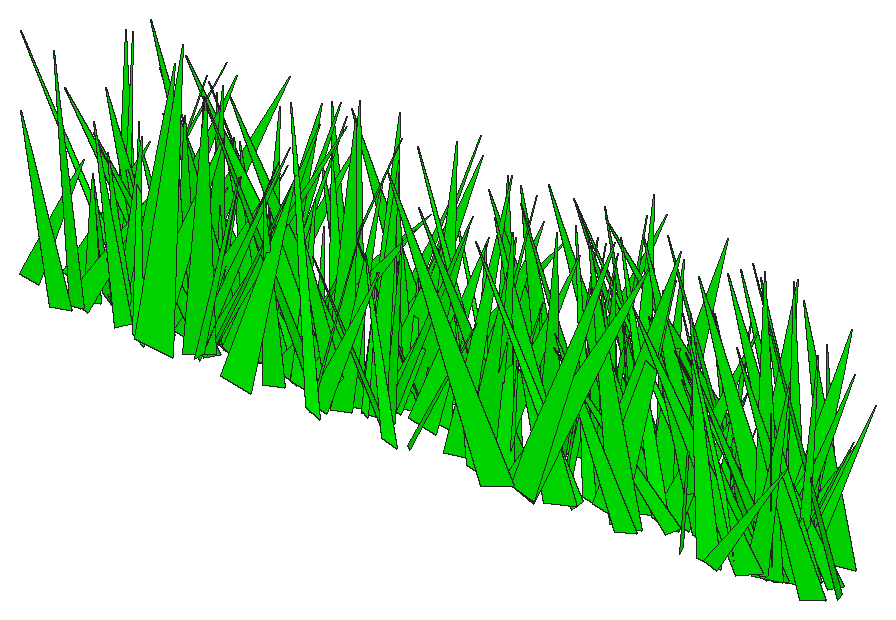
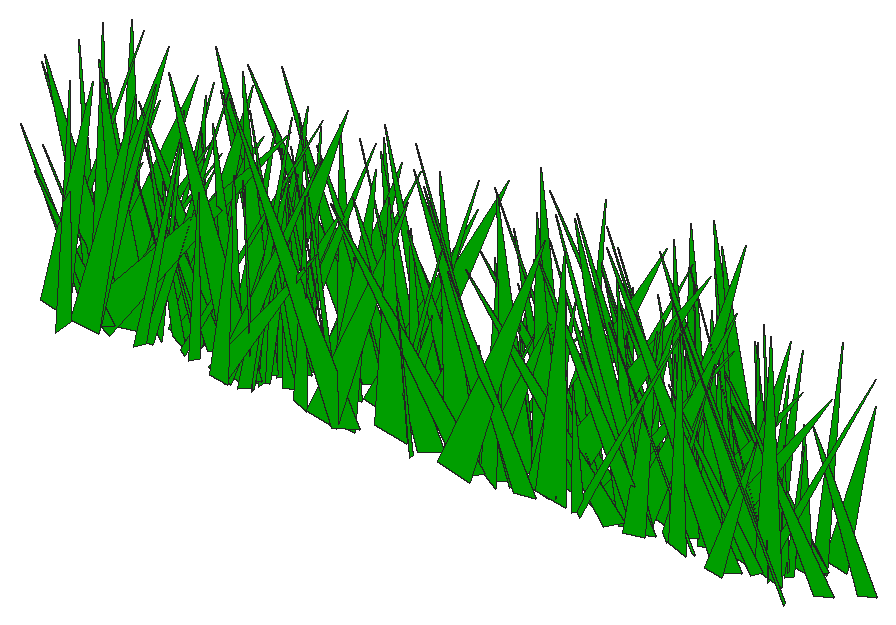
# SketchUp Ruby script. Lengths in inches.
U = 1.inch
M = Sketchup.active_model
def pt(a) = Geom::Point3d.new(a.map { |v| v * U })
def face(e, loops, mat)
  f = e.add_face(loops[0].map { |a| pt(a) })
  loops[1..].each { |l| e.add_face(l.map { |a| pt(a) }).erase! }
  f.material = f.back_material = mat if mat
  f
end
# faces: each face lists its corners as indices into pts; further lists are holes
def faces(e, pts, list, mat = nil) = list.each { |f| face(e, (f[0].is_a?(Array) ? f : [f]).map { |l| l.map { |i| pts[i] } }, mat) }
# xy, xz, yz: faces in a plane at the given z, y or x. An outline is a flat list of corners, or four numbers for a rectangle; further outlines are holes
def ring(l) = l.size == 4 ? [[l[0], l[1]], [l[2], l[1]], [l[2], l[3]], [l[0], l[3]]] : l.each_slice(2).to_a
def flat(e, list, mat, &to3) = list.each { |f| face(e, (f[0].is_a?(Array) ? f : [f]).map { |l| ring(l).map { |u, v| to3.(u, v) } }, mat) }
def xy(e, z, list, mat = nil) = flat(e, list, mat) { |x, y| [x, y, z] }
def xz(e, y, list, mat = nil) = flat(e, list, mat) { |x, z| [x, y, z] }
def yz(e, x, list, mat = nil) = flat(e, list, mat) { |y, z| [x, y, z] }
def lines(e, pts, list) = list.each { |a, b| e.add_line(pt(pts[a]), pt(pts[b])) }
# prism: a flat outline (further loops are holes) pulled along v
def prism(e, loops, v, mat = nil)
  f = face(e, loops, mat); d = Geom::Vector3d.new(v.map { |x| x * U })
  f.pushpull(f.normal.samedirection?(d) ? d.length : -d.length)
end
def box(e, o, s, mat = nil) = prism(e, [[o, [o[0] + s[0], o[1], o[2]], [o[0] + s[0], o[1] + s[1], o[2]], [o[0], o[1] + s[1], o[2]]]], [0, 0, s[2]], mat)
def at(x, y, z, deg = 0) = Geom::Transformation.translation(pt([x, y, z])) * Geom::Transformation.rotation(ORIGIN, Z_AXIS, deg.degrees)
def axes(o, x, y, z) = Geom::Transformation.new([*x, 0, *y, 0, *z, 0, *pt(o).to_a, 1])
def part(name) = M.definitions.add(name)
# library, detail: a bought-in or finely detailed component or shape, given as its bounding box
def library(name, o, s) = part(name).tap { |d| box(d.entities, o, s) }
def detail(e, o, s) = box(e.add_group.entities, o, s)
def put(e, d, t, mat = nil) = e.add_instance(d, t).tap { |i| i.material = mat if mat }
def group(e, t, mat = nil) = e.add_group.tap { |g| g.transformation = t; g.material = mat if mat }.entities
root = M.entities
M.materials.add("[0065_Lime]").color = [0, 255, 0]
c1 = part("fur_instance\#9")
p = [[0.8125,0,1.79],[0.67,-0.02,1.48],[0,-0.11,0],[0,0.11,0]]
faces(c1.entities,p,[[0,1,2,3]])
put(root,c1,axes([46.01,26.64,1.48],[0.39312,0.7455,1.32268],[-5.34892,0.11187,-1.06093],[-1.47663,-0.20675,4.19524]),"[0065_Lime]")
put(root,c1,axes([43.41,27.83,1.48],[1.65186,-0.62517,0.32117],[4.35522,0.21232,-0.97179],[0.99087,0.10897,3.73597]),"[0065_Lime]")
put(root,c1,axes([48.13,28.89,1.48],[-7.52684,0.16689,0.34184],[-1.24991,-1.03405,-1.29256],[0.15794,-0.2299,6.06191]),"[0065_Lime]")
put(root,c1,axes([46.45,27.2,1.48],[5.228,0.61413,2.31199],[-4.08637,0.83396,-1.30923],[-3.23754,-0.0609,5.38591]),"[0065_Lime]")
put(root,c1,axes([44.8125,28.98,1.48],[1.38787,0.72801,0.30258],[-4.98253,0.1713,1.31015],[1.46775,-0.10687,4.16142]),"[0065_Lime]")
put(root,c1,axes([46.98,28.53,1.48],[-3.31547,-0.39766,0.2806],[2.50986,-0.4424,-1.3872],[1.35212,-0.15388,3.26305]),"[0065_Lime]")
put(root,c1,axes([46.74,27.85,1.48],[2.77219,-0.52959,0.05829],[3.63715,0.37908,0.95828],[-0.99022,-0.09025,3.68301]),"[0065_Lime]")
put(root,c1,axes([47.58,29.18,1.48],[3.7097,0.99816,0.96893],[-6.88972,0.54666,-1.41749],[-2.09988,-0.03022,6.36253]),"[0065_Lime]")
put(root,c1,axes([47.47,29.06,1.48],[7.27811,-0.03007,2.93238],[1.38499,1.07577,-1.90478],[-3.33524,0.38111,5.60801]),"[0065_Lime]")
put(root,c1,axes([47.28,28.45,1.48],[-3.43906,-0.38807,0.41174],[2.028,-0.42111,-2.09235],[1.94182,-0.2475,2.91443]),"[0065_Lime]")
put(root,c1,axes([51.33,28.52,1.48],[-4.39004,0.70928,0.42442],[-4.77976,-0.5454,-2.16923],[-1.70433,-0.2974,4.99035]),"[0065_Lime]")
put(root,c1,axes([48.93,27.16,1.48],[4.57076,-0.57513,1.47257],[3.58658,0.68821,1.64116],[-2.67698,-0.05995,4.71313]),"[0065_Lime]")
put(root,c1,axes([46.08,27.49,1.48],[2.87351,0.50232,0.47351],[-3.35058,0.32902,1.75707],[1.3754,-0.24794,3.29108]),"[0065_Lime]")
put(root,c1,axes([49.69,30.24,1.48],[1.38702,-0.55697,1.32072],[3.87115,0.26565,1.06413],[-1.83349,0.13954,3.24587]),"[0065_Lime]")
put(root,c1,axes([48.87,27.45,1.48],[4.10355,-0.56754,0.67476],[3.56105,0.57072,1.75647],[-2.07844,-0.14269,4.34161]),"[0065_Lime]")
put(root,c1,axes([49.8,28.66,1.48],[2.54566,-1.01051,0.19163],[6.7882,0.34894,1.99328],[-2.3856,-0.08541,5.87635]),"[0065_Lime]")
put(root,c1,axes([45.73,30.47,1.48],[8.45305,0.14888,0.4382],[-1.1567,1.1555,1.60801],[-0.2736,-0.28534,6.74047]),"[0065_Lime]")
put(root,c1,axes([46.34,27.38,1.48],[3.2485,0.73838,0.04164],[-5.05982,0.43722,1.38144],[1.41874,-0.13138,4.83145]),"[0065_Lime]")
put(root,c1,axes([48.69,27.67,1.48],[4.18985,-0.68322,0.37128],[4.74827,0.58969,0.90814],[-1.14132,-0.05482,5.14118]),"[0065_Lime]")
put(root,c1,axes([50.78,27.65,1.48],[0.26537,0.70157,0.60757],[-4.81039,0.06703,-1.20343],[-1.53167,-0.08896,3.8848]),"[0065_Lime]")
put(root,c1,axes([50.18,26.6,1.48],[-6.18792,0.38686,1.2003],[-1.93536,-0.83601,2.42741],[2.45182,0.31645,4.94541]),"[0065_Lime]")
put(root,c1,axes([47.89,28.625,1.48],[8.27291,0.08504,1.06897],[-0.85805,1.15145,1.32436],[-1.16491,-0.24423,6.61602]),"[0065_Lime]")
put(root,c1,axes([53.44,27.49,1.48],[-3.93536,-0.65854,0.75026],[4.42389,-0.43921,2.43495],[-1.80101,0.36012,4.34166]),"[0065_Lime]")
put(root,c1,axes([48.18,29.23,1.48],[3.92831,0.46909,0.80178],[-3.34864,0.4523,1.98801],[0.95001,-0.34541,3.69209]),"[0065_Lime]")
put(root,c1,axes([49.65,27.41,1.48],[-1.32694,-1.12189,2.3141],[8.29308,-0.25541,-1.00283],[1.75012,0.35964,6.50656]),"[0065_Lime]")
put(root,c1,axes([50.09,28.35,1.48],[7.90295,-0.24361,1.86389],[0.99583,1.11613,2.09444],[-2.69527,-0.30191,6.23905]),"[0065_Lime]")
put(root,c1,axes([51.01,28.39,1.48],[3.61281,-0.64631,0.56121],[4.41092,0.51507,1.08876],[-1.47479,-0.04277,4.63117]),"[0065_Lime]")
put(root,c1,axes([48.38,28.74,1.48],[6.52384,-0.79979,0.80681],[5.77574,0.89755,-1.08577],[0.14481,0.23279,6.95813]),"[0065_Lime]")
put(root,c1,axes([51.08,28.69,1.48],[-3.06533,-0.95922,0.21111],[6.60434,-0.42634,-1.464],[1.74607,-0.07137,5.90806]),"[0065_Lime]")
put(root,c1,axes([51.12,26.47,1.48],[-2.83193,1.23815,1.54157],[-8.8212,-0.43803,1.06697],[1.84876,-0.19341,7.45235]),"[0065_Lime]")
put(root,c1,axes([53.14,29.13,1.48],[-5.98468,-0.162,1.22381],[1.57057,-0.81583,1.46278],[1.06121,0.2938,4.73681]),"[0065_Lime]")
put(root,c1,axes([52.08,29.66,1.48],[-4.88687,-0.46951,2.98277],[4.57373,-0.70654,1.23133],[1.9214,0.48771,4.65525]),"[0065_Lime]")
put(root,c1,axes([54.18,28.22,1.48],[-5.84031,-1.01171,1.45789],[7.41729,-0.80411,0.96127],[0.18511,0.30055,7.47945]),"[0065_Lime]")
put(root,c1,axes([54.8,28.91,1.48],[-4.56462,-0.87505,1.20839],[6.34569,-0.58447,1.67764],[-0.84761,0.33672,6.05221]),"[0065_Lime]")
put(root,c1,axes([50.42,27,1.48],[-0.24952,1.03081,0.55328],[-7.06553,-0.06057,1.67324],[2.08688,-0.08183,5.73124]),"[0065_Lime]")
put(root,c1,axes([52.09,28.16,1.48],[6.81858,0.01238,2.31874],[-0.60751,1.02055,0.99947],[-2.78654,-0.19221,5.456]),"[0065_Lime]")
put(root,c1,axes([49.15,29.9,1.48],[5.34224,0.95231,1.83705],[-7.02981,0.6304,2.57542],[1.26967,-0.51655,6.52986]),"[0065_Lime]")
put(root,c1,axes([52.4375,28.68,1.48],[-4.88319,-1.12671,0.44116],[7.40558,-0.66549,-2.71728],[3.12153,-0.18374,7.13667]),"[0065_Lime]")
put(root,c1,axes([53.08,28.45,1.48],[3.98186,-0.48678,0.76105],[3.24055,0.57216,1.04494],[-1.54099,-0.05461,4.16396]),"[0065_Lime]")
put(root,c1,axes([56.91,29.1,1.48],[-6.95745,0.30583,0.08805],[-2.03912,-0.89576,-2.3518],[-0.76845,-0.39196,5.4434]),"[0065_Lime]")
put(root,c1,axes([52.93,27.25,1.48],[5.59851,-1.057,0.00119],[7.29692,0.76319,1.85184],[-1.82716,-0.19084,7.3991]),"[0065_Lime]")
put(root,c1,axes([51.31,29.54,1.48],[6.37022,0.00424,0.20532],[-0.08097,0.87705,1.05461],[-0.24097,-0.18249,5.07322]),"[0065_Lime]")
put(root,c1,axes([52.99,27.8,1.48],[5.14899,0.24899,1.02619],[-1.52147,0.73783,-0.94792],[-1.55455,0.10259,4.32671]),"[0065_Lime]")
put(root,c1,axes([54.27,29.82,1.48],[-3.4233,-0.80208,0.13917],[5.58242,-0.47593,-1.05904],[1.20324,-0.07391,5.3094]),"[0065_Lime]")
put(root,c1,axes([51.51,28.06,1.48],[4.63741,-0.68007,0.24378],[4.77606,0.63053,-1.17118],[0.83815,0.16981,5.32496]),"[0065_Lime]")
put(root,c1,axes([57.29,29.78,1.48],[-7.49559,-0.24369,0.29526],[1.77152,-1.0348,1.13702],[0.03232,0.20288,6.15392]),"[0065_Lime]")
put(root,c1,axes([53.03,27.13,1.48],[6.13237,-0.24377,0.81897],[1.4504,0.85326,1.32493],[-1.38553,-0.18574,5.01174]),"[0065_Lime]")
put(root,c1,axes([55.07,28.26,1.48],[1.99362,0.82632,1.38089],[-5.87868,0.32836,-0.96863],[-1.70411,-0.16603,4.95697]),"[0065_Lime]")
put(root,c1,axes([56.12,28.57,1.48],[0.6473,0.87919,1.85304],[-6.31254,0.18336,-1.45628],[-2.11875,-0.27771,4.9049]),"[0065_Lime]")
put(root,c1,axes([52.63,27.53,1.48],[8.08582,-0.06991,0.57361],[0.15516,1.03622,2.78472],[-0.84896,-0.47645,5.97223]),"[0065_Lime]")
put(root,c1,axes([59.64,28.28,1.48],[-4.89287,1.11429,0.32486],[-7.51497,-0.62864,-2.63499],[-2.56277,-0.28403,7.10652]),"[0065_Lime]")
put(root,c1,axes([52.71,27.37,1.48],[8.05292,0.26091,1.23659],[-2.3301,1.02904,2.76437],[-0.57396,-0.51689,6.12752]),"[0065_Lime]")
put(root,c1,axes([55.54,28.375,1.48],[5.14855,0.90171,0.48123],[-5.99065,0.70891,-2.10489],[-2.37504,0.16659,6.35243]),"[0065_Lime]")
put(root,c1,axes([53.25,27.68,1.48],[6.91534,-0.15036,0.22191],[0.99941,0.95558,1.09031],[-0.46974,-0.18052,5.58657]),"[0065_Lime]")
put(root,c1,axes([59.17,27.43,1.48],[-7.44723,-0.50567,0.47766],[3.64612,-1.03142,1.02364],[-0.02633,0.1951,6.6495]),"[0065_Lime]")
put(root,c1,axes([54.53,29.3,1.48],[-0.3354,-1.21438,1.28591],[8.49047,-0.10194,-1.76065],[2.25808,0.20292,6.8111]),"[0065_Lime]")
put(root,c1,axes([56.52,28.0625,1.48],[5.40285,0.01826,2.23878],[-1.04479,0.80128,1.44931],[-2.54963,-0.28966,4.15024]),"[0065_Lime]")
put(root,c1,axes([54.06,28,1.48],[6.8817,0.62894,1.60068],[-4.87368,0.92059,1.74264],[-0.3913,-0.40505,6.44608]),"[0065_Lime]")
put(root,c1,axes([54.38,29.42,1.48],[7.60058,0.52779,1.797],[-4.26964,1.02677,1.84314],[-0.8711,-0.42751,6.64526]),"[0065_Lime]")
put(root,c1,axes([52.98,27.55,1.48],[8.95041,-0.29126,0.18647],[2.08197,1.23985,-1.22578],[0.11978,0.21353,7.37184]),"[0065_Lime]")
put(root,c1,axes([53.92,29.52,1.48],[5.14334,0.80195,0.77013],[-5.72698,0.68065,1.55621],[0.81808,-0.27705,6.05241]),"[0065_Lime]")
put(root,c1,axes([54.9,28.9,1.48],[8.2794,-0.03942,1.42426],[0.90443,1.1044,-2.45423],[-1.52532,0.44085,6.27561]),"[0065_Lime]")
put(root,c1,axes([57.04,27.08,1.48],[3.18206,-0.73976,0.77628],[5.13718,0.46604,0.94903],[-1.49515,0.02686,4.91288]),"[0065_Lime]")
put(root,c1,axes([55.73,26.16,1.48],[-1.14938,1.02905,0.12434],[-7.06423,-0.16148,1.57532],[1.93655,0.02172,5.82034]),"[0065_Lime]")
put(root,c1,axes([57.32,29.71,1.48],[-3.14318,0.39124,0.59405],[-2.5294,-0.44794,1.03062],[1.37395,0.0704,3.25634]),"[0065_Lime]")
put(root,c1,axes([60.89,27.79,1.48],[-2.47953,-1.12851,1.67586],[7.88845,-0.22807,2.57602],[-2.55258,0.3914,6.33299]),"[0065_Lime]")
put(root,c1,axes([57.87,27.74,1.48],[-4.24002,0.52215,1.21443],[-3.36974,-0.63028,1.29652],[2.16378,0.04162,4.39884]),"[0065_Lime]")
put(root,c1,axes([58.875,29.59,1.48],[2.1151,1.06656,1.4087],[-7.61446,0.33594,-0.95862],[-1.62202,-0.18627,6.33713]),"[0065_Lime]")
put(root,c1,axes([58.58,29.54,1.48],[-4.48414,-0.05298,1.57068],[-0.28031,-0.65124,-1.26552],[1.94736,-0.21573,3.4346]),"[0065_Lime]")
put(root,c1,axes([59.7,29.42,1.48],[2.01355,0.77076,2.07147],[-5.66349,0.37259,-1.00305],[-2.1206,-0.26322,4.64575]),"[0065_Lime]")
put(root,c1,axes([59.74,26.3,1.48],[-8.53543,0.46026,1.51348],[-2.52466,-1.17952,2.59906],[2.79583,0.34001,6.96751]),"[0065_Lime]")
put(root,c1,axes([59.79,28.03,1.48],[-4.87525,0.79032,0.41269],[-5.41076,-0.68069,1.38913],[1.6169,0.10511,5.89289]),"[0065_Lime]")
put(root,c1,axes([60.34,27.38,1.48],[0.78176,-0.7928,0.92803],[5.55813,0.14604,1.08282],[-1.49706,0.12822,4.50482]),"[0065_Lime]")
put(root,c1,axes([55.45,29.62,1.48],[3.69795,0.83838,0.97094],[-5.41072,0.36332,3.12248],[2.78321,-0.40761,4.78023]),"[0065_Lime]")
put(root,c1,axes([59.76,28.7,1.48],[3.56061,1.15935,0.65761],[-8.11599,0.51269,-1.21256],[-1.69012,-0.01952,7.20814]),"[0065_Lime]")
put(root,c1,axes([57.18,28.14,1.48],[8.78679,0.04487,0.71432],[-0.13824,1.2165,-1.43522],[-0.92414,0.24461,7.00652]),"[0065_Lime]")
put(root,c1,axes([56.8,28.08,1.48],[3.16881,-0.84147,1.04562],[5.59461,0.31491,-2.72608],[2.49256,0.36295,4.78944]),"[0065_Lime]")
put(root,c1,axes([59.64,28.19,1.48],[6.00616,-0.99073,0.94652],[6.89846,0.85959,1.18667],[-1.86445,-0.01106,7.43979]),"[0065_Lime]")
put(root,c1,axes([59.51,26.49,1.48],[6.12792,0.26594,0.80516],[-1.47015,0.83178,-1.80278],[-1.54926,0.26257,4.89545]),"[0065_Lime]")
put(root,c1,axes([62.66,29,1.48],[-1.55399,0.73323,0.6535],[-5.13807,-0.18298,-1.20454],[-1.21395,-0.16415,4.26169]),"[0065_Lime]")
put(root,c1,axes([63.49,30.3,1.48],[1.42616,-1.05769,2.52391],[7.46644,0.3464,2.07286],[-3.24611,0.33207,5.8767]),"[0065_Lime]")
put(root,c1,axes([59.61,26.77,1.48],[2.12493,-0.61698,1.07974],[4.5004,0.24065,-1.25209],[0.88726,0.25697,3.76502]),"[0065_Lime]")
put(root,c1,axes([60.58,27.16,1.48],[5.11562,0.82897,0.14497],[-5.70325,0.70283,-1.5131],[-1.51916,0.15291,6.16868]),"[0065_Lime]")
put(root,c1,axes([63.44,26.69,1.48],[-4.75103,-0.21791,0.37727],[1.60323,-0.60572,1.63504],[-0.22272,0.28818,3.72189]),"[0065_Lime]")
put(root,c1,axes([61.41,28.6,1.48],[-4.47976,1.13271,0.65387],[-7.79437,-0.63785,1.694],[2.20766,0.04651,7.30764]),"[0065_Lime]")
put(root,c1,axes([61.51,27.58,1.48],[-4.11415,0.22093,1.26368],[-0.92549,-0.59106,1.46913],[2.00725,0.18031,3.26747]),"[0065_Lime]")
put(root,c1,axes([59.9,30.04,1.48],[2.89391,0.80162,0.49148],[-5.67724,0.38655,0.99142],[0.82348,-0.15216,5.1079]),"[0065_Lime]")
put(root,c1,axes([63.53,29.05,1.48],[-5.21985,-0.26238,0.02544],[1.81394,-0.71545,-1.00304],[0.44405,-0.16171,4.39641]),"[0065_Lime]")
put(root,c1,axes([61.91,29.31,1.48],[-3.50641,-0.45996,0.70406],[2.85772,-0.49595,-1.44024],[1.81579,-0.10767,3.62625]),"[0065_Lime]")
put(root,c1,axes([61.97,29.87,1.48],[7.09496,-0.57575,0.99658],[3.01346,0.90969,3.41594],[-3.03451,-0.44277,5.72233]),"[0065_Lime]")
put(root,c1,axes([61.92,27.66,1.48],[4.61694,0.90954,0.9321],[-6.36337,0.66776,-0.97973],[-1.64846,-0.03028,6.39252]),"[0065_Lime]")
put(root,c1,axes([62.74,29.11,1.48],[-2.99621,0.39994,0.42796],[-2.56057,-0.41587,1.16165],[1.34947,0.09889,3.15438]),"[0065_Lime]")
put(root,c1,axes([63.84,26.28,1.48],[-4.62789,0.4755,0.0564],[-3.21106,-0.62204,1.40093],[1.07003,0.18989,4.44798]),"[0065_Lime]")
put(root,c1,axes([62.48,28.04,1.48],[-4.39996,-0.48608,1.56876],[3.02039,-0.67385,-1.39136],[2.56181,-0.04038,4.3348]),"[0065_Lime]")
put(root,c1,axes([60.85,29.73,1.48],[9.22928,0.19884,1.22774],[-1.72829,1.27395,1.68243],[-1.13734,-0.32236,7.40625]),"[0065_Lime]")
put(root,c1,axes([62.02,28.69,1.48],[1.15081,0.67309,0.65078],[-4.70141,0.12545,1.15287],[1.21717,-0.15182,3.83774]),"[0065_Lime]")
put(root,c1,axes([61.26,29.46,1.48],[5.96403,-0.8237,1.68685],[6.21747,0.78505,-1.69892],[0.07629,0.41345,6.58661]),"[0065_Lime]")
put(root,c1,axes([62.54,29.13,1.48],[-1.74674,-1.07994,0.05926],[7.0375,-0.22895,-2.56472],[3.08956,-0.08905,5.87551]),"[0065_Lime]")
put(root,c1,axes([62.22,28.39,1.48],[7.45606,-0.29233,0.25308],[1.98959,1.03233,1.17477],[-0.68289,-0.18409,6.18595]),"[0065_Lime]")
put(root,c1,axes([64.33,28.83,1.48],[-4.93218,0.95413,1.78389],[-6.65287,-0.75034,1.27767],[2.57964,-0.11085,6.70584]),"[0065_Lime]")
put(root,c1,axes([66.46,28.92,1.48],[-0.24645,-0.56376,0.60256],[3.90422,-0.00232,0.98368],[-1.18406,0.10968,3.11809]),"[0065_Lime]")
put(root,c1,axes([64,28.31,1.48],[-0.41496,0.94979,0.29257],[-6.51221,-0.06983,1.48489],[1.84587,-0.03284,5.30446]),"[0065_Lime]")
put(root,c1,axes([67.55,28.78,1.48],[-8.18823,0.19865,1.4565],[-1.72631,-1.15239,-1.15458],[1.49153,-0.24324,6.65961]),"[0065_Lime]")
put(root,c1,axes([65.68,30.39,1.48],[4.00759,0.0919,1.26202],[-1.10109,0.56887,0.92531],[-1.2738,-0.20259,3.1707]),"[0065_Lime]")
put(root,c1,axes([67.85,28.89,1.48],[-6.64557,0.23882,0.58207],[-1.36451,-0.8898,1.92564],[1.24042,0.30065,5.23674]),"[0065_Lime]")
put(root,c1,axes([64.71,26.49,1.48],[4.83906,0.03129,0.24],[-0.11992,0.64777,-1.23033],[-0.34967,0.2109,3.74332]),"[0065_Lime]")
put(root,c1,axes([69.62,26.27,1.48],[-0.4875,1.21552,1.08315],[-8.09173,0.00882,-2.74141],[-3.33541,-0.19906,6.49239]),"[0065_Lime]")
put(root,c1,axes([62.64,30.04,1.48],[5.40906,-0.73557,0.24988],[4.92252,0.69091,-2.35008],[1.80704,0.3197,5.65383]),"[0065_Lime]")
put(root,c1,axes([69.45,27.99,1.48],[-3.91466,-0.9082,0.16303],[6.38544,-0.53774,1.06658],[-1.01969,0.11921,6.05316]),"[0065_Lime]")
put(root,c1,axes([67.51,29.45,1.48],[2.22423,1.12947,0.03787],[-7.9163,0.30898,-1.16583],[-1.3936,0.0475,6.6829]),"[0065_Lime]")
put(root,c1,axes([67.86,26.78,1.48],[-4.02814,0.30472,0.37302],[-1.93852,-0.54913,1.18133],[1.07479,0.15162,3.5287]),"[0065_Lime]")
put(root,c1,axes([65.25,29.59,1.48],[3.22894,-0.79455,2.46855],[6.3745,0.342,-1.82815],[0.74085,0.52034,4.971]),"[0065_Lime]")
put(root,c1,axes([67.36,27.9,1.48],[-5.05395,0.56585,0.90242],[-3.57052,-0.71225,1.73478],[2.16752,0.14611,4.96181]),"[0065_Lime]")
put(root,c1,axes([66.625,27.19,1.48],[6.70628,0.90979,0.56499],[-6.2616,0.93944,-1.51556],[-1.78734,0.12245,7.42938]),"[0065_Lime]")
put(root,c1,axes([66.94,27.9375,1.48],[7.85998,0.43558,1.12373],[-2.79176,1.10832,-1.4757],[-1.92962,0.17074,6.71235]),"[0065_Lime]")
put(root,c1,axes([70.53,30.27,1.48],[-2.12604,-1.0567,0.50328],[7.42861,-0.27729,1.25373],[-1.32281,0.14112,6.23181]),"[0065_Lime]")
put(root,c1,axes([67.24,29.375,1.48],[4.70986,0.15379,0.8766],[-1.34419,0.64902,0.96313],[-0.74318,-0.19927,3.81339]),"[0065_Lime]")
put(root,c1,axes([67.58,27.77,1.48],[-0.51986,-1.08377,0.69763],[7.60409,-0.09525,-1.20926],[1.54898,0.10386,6.17048]),"[0065_Lime]")
put(root,c1,axes([69.77,30.14,1.48],[1.90416,-1.08438,1.27746],[7.68399,0.30556,1.11312],[-1.7249,0.1641,6.36886]),"[0065_Lime]")
put(root,c1,axes([68.27,28.17,1.48],[7.96335,-0.68355,0.24754],[4.12527,0.98887,3.69444],[-2.59579,-0.52546,6.63067]),"[0065_Lime]")
put(root,c1,axes([69.24,27.16,1.48],[-2.60949,0.6813,0.00674],[-4.71619,-0.35698,1.03579],[1.12513,0.0838,4.35736]),"[0065_Lime]")
put(root,c1,axes([69.4,27.45,1.48],[3.87697,-0.14184,0.87911],[0.56219,0.53549,1.25469],[-1.3678,-0.18194,3.00748]),"[0065_Lime]")
put(root,c1,axes([70.0625,29.16,1.48],[-3.2817,-0.51877,0.672],[3.5066,-0.47479,-0.95181],[1.41996,-0.02646,3.90357]),"[0065_Lime]")
put(root,c1,axes([67.98,27.83,1.48],[4.04067,0.85802,1.26718],[-6.25375,0.51394,1.53312],[0.77626,-0.32583,5.75513]),"[0065_Lime]")
put(root,c1,axes([72.64,26.68,1.48],[0.14817,1.16562,0.34287],[-7.9503,0.03705,-1.94763],[-2.40431,-0.05069,6.46135]),"[0065_Lime]")
put(root,c1,axes([73.25,27.04,1.48],[-7.25624,0.23932,0.89509],[-1.96936,-0.9686,-1.88519],[0.48287,-0.35407,5.76218]),"[0065_Lime]")
put(root,c1,axes([70.71,28.26,1.48],[-4.40764,-0.98146,1.0435],[6.58982,-0.64435,-1.89112],[2.64669,-0.03015,6.44636]),"[0065_Lime]")
put(root,c1,axes([71.99,29.91,1.48],[4.83844,0.54238,1.83027],[-3.70305,0.74759,-0.94667],[-2.49985,-0.05763,4.94478]),"[0065_Lime]")
put(root,c1,axes([74.56,27.72,1.48],[-7.4647,-0.48621,1.46158],[3.86397,-0.99536,1.96164],[0.52051,0.41622,6.39854]),"[0065_Lime]")
put(root,c1,axes([70.78,29.08,1.48],[8.5998,-0.23614,1.43037],[0.74325,1.1196,3.23696],[-2.316,-0.51753,6.35006]),"[0065_Lime]")
put(root,c1,axes([71.7,28.15,1.48],[7.39284,0.33709,1.45028],[-1.60225,1.0112,-2.47178],[-2.52319,0.34553,5.81887]),"[0065_Lime]")
put(root,c1,axes([69.29,30.25,1.48],[6.49197,-0.87366,0.75193],[6.25527,0.87957,-1.48812],[0.61841,0.27461,7.15873]),"[0065_Lime]")
put(root,c1,axes([71.46,28.73,1.48],[7.02328,-0.06779,1.6131],[0.85287,1.00471,-1.04209],[-1.85421,0.20537,5.63067]),"[0065_Lime]")
put(root,c1,axes([73.41,27.65,1.48],[-7.33614,0.37282,1.8212],[-2.19066,-1.06772,1.48553],[2.69319,0.14704,6.16924]),"[0065_Lime]")
put(root,c1,axes([70.77,26.44,1.48],[5.70314,0.93016,1.20085],[-6.78151,0.77841,1.10547],[0.09231,-0.28167,7.02069]),"[0065_Lime]")
put(root,c1,axes([76.02,28.3,1.48],[-0.34668,1.16289,3.01603],[-8.62351,0.11903,-2.19375],[-2.80554,-0.50957,6.37034]),"[0065_Lime]")
put(root,c1,axes([76.03,30.01,1.48],[-6.65257,-0.62246,0.97914],[4.58928,-0.90845,1.27844],[0.10145,0.27782,6.37424]),"[0065_Lime]")
put(root,c1,axes([76.31,30.06,1.48],[-3.43682,-0.59958,0.80979],[4.13007,-0.38394,2.07165],[-1.46304,0.32463,3.94586]),"[0065_Lime]")
put(root,c1,axes([73.125,28.97,1.48],[-3.86138,-0.83869,1.05536],[5.62187,-0.57234,-1.6314],[2.38789,-0.00876,5.54744]),"[0065_Lime]")
put(root,c1,axes([74.37,29.37,1.48],[-5.38327,-0.57449,0.73209],[3.81244,-0.75789,-1.38028],[1.72915,-0.11753,5.32241]),"[0065_Lime]")
put(root,c1,axes([74.03,28.29,1.48],[-4.89731,0.65,0.39399],[-4.24036,-0.66459,1.86657],[1.91084,0.19108,5.15188]),"[0065_Lime]")
put(root,c1,axes([74.75,30.16,1.48],[-7.56855,-0.62904,1.11517],[4.00684,-1.05971,-2.03734],[2.42165,-0.21258,6.85631]),"[0065_Lime]")
put(root,c1,axes([73.02,28.91,1.48],[8.00536,0.53053,1.29765],[-3.08937,1.10427,-2.51813],[-2.69358,0.3102,6.74479]),"[0065_Lime]")
put(root,c1,axes([70.6,26.49,1.48],[3.93557,1.08245,1.46137],[-7.64869,0.44889,2.48718],[2.01643,-0.40995,6.58211]),"[0065_Lime]")
put(root,c1,axes([75.23,29.86,1.48],[0.14951,-0.95437,0.6044],[6.71649,0.03968,1.00017],[-1.25271,0.09884,5.4346]),"[0065_Lime]")
put(root,c1,axes([76.27,26.52,1.48],[-1.80974,0.73582,0.26753],[-5.04008,-0.23021,-1.34093],[-1.45827,-0.1175,4.30251]),"[0065_Lime]")
put(root,c1,axes([74.38,29.47,1.48],[-4.88612,-0.36659,1.07541],[1.95527,-0.67844,-1.8716],[2.17505,-0.21363,4.09833]),"[0065_Lime]")
put(root,c1,axes([74.67,29.72,1.48],[6.45953,0.23507,2.0805],[-0.37795,0.89535,-2.61348],[-3.03277,0.3891,4.75697]),"[0065_Lime]")
put(root,c1,axes([77.77,27.84,1.48],[-3.64545,0.52778,0.29446],[-3.28566,-0.40921,-2.33658],[-1.85547,-0.31231,3.55909]),"[0065_Lime]")
put(root,c1,axes([75.99,26.875,1.48],[1.34755,1.11394,1.46472],[-7.88605,0.2414,-1.35152],[-1.97387,-0.20397,6.39958]),"[0065_Lime]")
put(root,c1,axes([74.83,28.79,1.48],[-6.448,0.88838,2.13132],[-6.01346,-0.97698,1.6085],[3.26706,-0.04492,7.1671]),"[0065_Lime]")
put(root,c1,axes([78.64,29.43,1.48],[-9.28261,-0.00678,0.24278],[-0.02698,-1.26465,-1.86533],[0.30113,-0.32219,7.31666]),"[0065_Lime]")
put(root,c1,axes([76.95,28.02,1.48],[-7.48328,0.56621,0.5191],[-3.68198,-1.01803,2.0895],[1.75691,0.27819,6.59001]),"[0065_Lime]")
put(root,c1,axes([76.02,30.31,1.48],[2.87808,-0.58675,0.68845],[3.99065,0.42152,1],[-1.49223,-0.00439,4.0021]),"[0065_Lime]")
put(root,c1,axes([76.23,29.15,1.48],[-4.68576,0.68628,0.42451],[-4.59976,-0.64866,1.54644],[1.72272,0.13471,5.28375]),"[0065_Lime]")
put(root,c1,axes([74,27.87,1.48],[1.06106,-1.23544,1.6223],[8.78764,0.07869,-1.79471],[2.01393,0.30754,6.97634]),"[0065_Lime]")
put(root,c1,axes([74.67,27.34,1.48],[-1.08811,1.05699,1.67996],[-7.45286,-0.22737,1.59976],[2.30267,-0.23644,5.97168]),"[0065_Lime]")
put(root,c1,axes([76.05,28.96,1.48],[4.44949,0.92869,0.47857],[-6.43026,0.62808,-1.28524],[-1.63631,0.05712,6.35197]),"[0065_Lime]")
put(root,c1,axes([75.27,29.52,1.48],[1.44692,1.18467,1.57238],[-8.53209,0.15026,1.40121],[1.42034,-0.30421,6.81538]),"[0065_Lime]")
put(root,c1,axes([79.33,28.41,1.48],[2.30347,-1.03442,2.8308],[7.57797,0.4583,1.53184],[-2.97957,0.36589,6.08439]),"[0065_Lime]")
put(root,c1,axes([77.88,29.61,1.48],[-4.69988,0.32191,1.18712],[-2.00398,-0.68759,0.99842],[1.83358,0.07362,4.13405]),"[0065_Lime]")
put(root,c1,axes([79.13,28.29,1.48],[-0.95614,-0.89318,0.74818],[6.33197,-0.10922,0.98469],[-1.07492,0.15108,5.13495]),"[0065_Lime]")
put(root,c1,axes([83.11,29.6,1.48],[-5.70179,-1.05499,0.21922],[6.8307,-0.70821,3.34304],[-3.12767,0.37657,6.90143]),"[0065_Lime]")
put(root,c1,axes([80.27,29.72,1.48],[-7.86598,-0.49981,0.80469],[3.40613,-1.10867,-1.04521],[1.42425,-0.10896,6.94381]),"[0065_Lime]")
put(root,c1,axes([79.04,26.76,1.48],[5.89463,0.30477,1.5739],[-1.36678,0.83323,-2.01973],[-2.56519,0.25639,4.69287]),"[0065_Lime]")
put(root,c1,axes([82.54,26.92,1.48],[-1.75383,1.00094,0.84537],[-6.60684,-0.16413,-2.55703],[-2.85841,-0.23478,5.39155]),"[0065_Lime]")
put(root,c1,axes([77.6,28.44,1.48],[0.89109,0.66962,0.91436],[-4.65314,0.06587,1.38398],[1.52336,-0.1905,3.69255]),"[0065_Lime]")
put(root,c1,axes([77.11,28.15,1.48],[3.17439,0.90359,0.44563],[-6.36225,0.42376,1.1939],[1.0826,-0.15913,5.7097]),"[0065_Lime]")
put(root,c1,axes([80.42,30.06,1.48],[-6.15039,-0.54836,0.51288],[3.43604,-0.82262,-2.2091],[1.95447,-0.27939,5.49763]),"[0065_Lime]")
put(root,c1,axes([80.14,29.08,1.48],[6.37743,-0.19927,2.46781],[0.38221,0.95428,1.92856],[-3.32709,-0.27234,4.9519]),"[0065_Lime]")
put(root,c1,axes([79.26,28.91,1.48],[5.46489,0.57965,0.64325],[-3.77174,0.75748,-1.67123],[-1.84814,0.1681,5.31277]),"[0065_Lime]")
put(root,c1,axes([80.63,26.59,1.48],[-5.03592,0.75413,0.71092],[-5.23946,-0.71776,0.95666],[1.45405,0.02547,5.90941]),"[0065_Lime]")
put(root,c1,axes([78.54,28.61,1.48],[5.73558,-0.04429,0.64371],[0.13352,0.79434,1.04432],[-0.84131,-0.17589,4.55423]),"[0065_Lime]")
put(root,c1,axes([79.16,28.48,1.48],[-0.42075,-0.65574,0.34695],[4.46948,-0.07424,-1.11556],[1.40819,0.0397,3.64437]),"[0065_Lime]")
put(root,c1,axes([80.1,27.8,1.48],[-2.09163,0.59216,0.40953],[-4.05867,-0.30214,0.92431],[1.24088,0.0099,3.71354]),"[0065_Lime]")
put(root,c1,axes([82.21,27.67,1.48],[-1.11912,-0.73526,0.46089],[5.05311,-0.12734,1.31086],[-1.47172,0.12187,4.15033]),"[0065_Lime]")
put(root,c1,axes([81.86,27.07,1.48],[-7.21918,-0.00618,1.50536],[-0.38346,-1.01925,-1.35696],[1.81105,-0.24045,5.71335]),"[0065_Lime]")
put(root,c1,axes([79.27,28.58,1.48],[4.80664,0.01167,0.45871],[-0.21499,0.66031,0.92779],[-0.52791,-0.16268,3.79871]),"[0065_Lime]")
put(root,c1,axes([83.45,28,1.48],[-6.38149,0.11557,0.17122],[-0.84261,-0.83482,-1.89688],[-0.10367,-0.3287,4.87787]),"[0065_Lime]")
put(root,c1,axes([83.95,27.29,1.48],[-4.537,-0.5915,0.85812],[4.26038,-0.56632,1.82294],[-0.82538,0.32817,4.69255]),"[0065_Lime]")
put(root,c1,axes([83.02,30,1.48],[-7.33488,0.33241,1.89082],[-2.91154,-1.02504,-1.43437],[1.58829,-0.34392,6.10261]),"[0065_Lime]")
put(root,c1,axes([84.01,27.3125,1.48],[-1.32853,1.20069,0.47086],[-8.26933,-0.15842,-1.90073],[-2.22854,-0.12794,6.77225]),"[0065_Lime]")
put(root,c1,axes([83.19,30.26,1.48],[-4.47734,0.79806,2.02407],[-6.17829,-0.61076,-0.97309],[0.52579,-0.38087,5.80159]),"[0065_Lime]")
put(root,c1,axes([81.37,29.2,1.48],[-1.72679,1.16722,0.773],[-8.22371,-0.26171,1.08699],[1.50755,-0.09065,6.81498]),"[0065_Lime]")
put(root,c1,axes([84.78,27.98,1.48],[-5.30199,0.87993,2.01684],[-6.73471,-0.69733,-1.51931],[0.07096,-0.43609,6.49895]),"[0065_Lime]")
put(root,c1,axes([80.78,26.51,1.48],[3.00644,-0.41744,0.51482],[2.9048,0.35857,-1.48099],[0.8877,0.24043,3.10261]),"[0065_Lime]")
put(root,c1,axes([83.34,27.11,1.48],[4.10067,1.17864,0.87856],[-8.12314,0.59586,-1.7005],[-2.353,-0.003,7.40163]),"[0065_Lime]")
put(root,c1,axes([81.76,28.45,1.48],[1.99789,0.54027,0.14682],[-3.72999,0.2647,0.94371],[0.9502,-0.09692,3.3958]),"[0065_Lime]")
put(root,c1,axes([83.4,28.98,1.48],[-6.90359,0.43291,3.43383],[-4.11323,-1.05637,-1.00874],[3.22398,-0.42073,6.06597]),"[0065_Lime]")
put(root,c1,axes([83.39,27.34,1.48],[4.78516,-0.00719,1.70895],[-0.54808,0.7045,1.11468],[-2.02886,-0.20727,3.72952]),"[0065_Lime]")
put(root,c1,axes([82.72,27.16,1.48],[2.82588,0.69511,2.14527],[-5.60168,0.36632,0.90478],[-0.2187,-0.40103,4.54488]),"[0065_Lime]")
put(root,c1,axes([85.95,26.89,1.48],[0.64433,0.97951,0.98405],[-6.48577,0.14997,-2.19254],[-2.82659,-0.12084,5.25523]),"[0065_Lime]")
put(root,c1,axes([86.06,28.29,1.48],[-3.74624,0.45917,0.97559],[-3.42288,-0.44093,-1.74233],[-0.63278,-0.33331,3.64897]),"[0065_Lime]")
put(root,c1,axes([85.15,29.83,1.48],[1.47103,1.00064,1.75555],[-7.17951,0.27209,-1.21649],[-1.95506,-0.24631,5.78821]),"[0065_Lime]")
put(root,c1,axes([86.66,27.8,1.48],[-9.07027,-0.18014,1.41826],[1.75462,-1.23008,2.18918],[1.26683,0.41396,7.12235]),"[0065_Lime]")
put(root,c1,axes([82.55,29.66,1.48],[0.41371,0.64826,0.2182],[-4.27804,0.03942,1.44276],[1.74745,-0.05698,3.48046]),"[0065_Lime]")
put(root,c1,axes([83.87,30.86,1.48],[-6.8572,-0.79726,0.37301],[4.38548,-0.80426,-4.26019],[3.62888,-0.53456,5.85326]),"[0065_Lime]")
put(root,c1,axes([83.77,29.04,1.48],[4.16371,-0.26883,0.38185],[1.65387,0.56085,1.29914],[-1.07014,-0.17918,3.49349]),"[0065_Lime]")
put(root,c1,axes([83.2,28.46,1.48],[-2.80573,1.12469,0.16361],[-7.50828,-0.38001,2.34156],[2.77996,0.10876,6.48935]),"[0065_Lime]")
put(root,c1,axes([82.93,28.39,1.48],[5.61898,0.53026,1.06971],[-3.98716,0.76537,1.14385],[-0.26924,-0.26789,5.3855]),"[0065_Lime]")
put(root,c1,axes([83.375,28.42,1.48],[4.83224,0.04655,0.25777],[-0.21241,0.64517,-1.26925],[-0.40624,0.21634,3.72978]),"[0065_Lime]")
put(root,c1,axes([84.13,28.36,1.48],[7.35615,-0.46438,0.96296],[2.59982,0.98023,2.69959],[-2.35883,-0.36783,5.97844]),"[0065_Lime]")
put(root,c1,axes([83.75,29.22,1.48],[5.71711,-0.13192,1.27997],[1.63213,0.69592,-2.41999],[-0.83287,0.45822,4.04386]),"[0065_Lime]")
